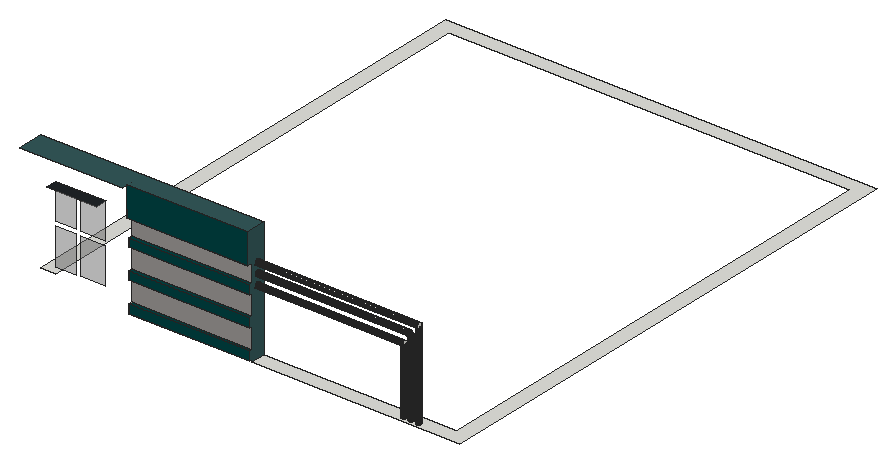
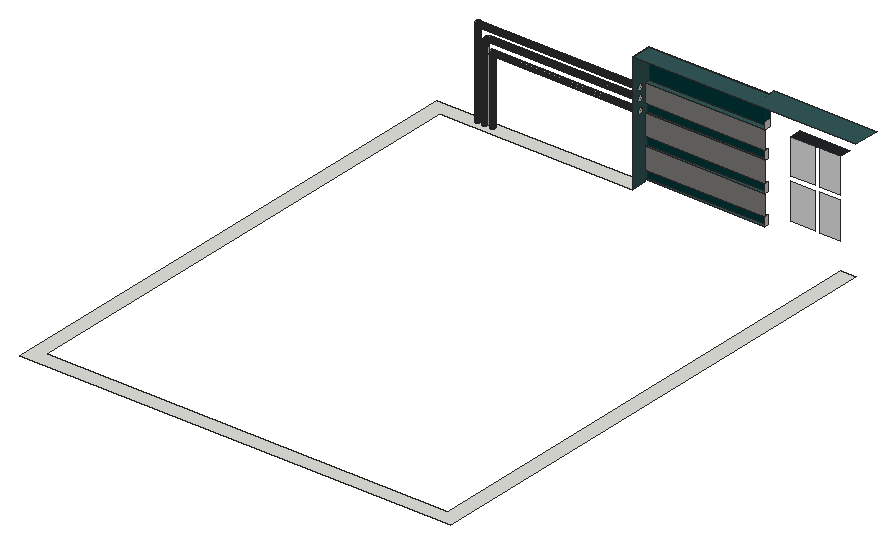
# SketchUp Ruby script. Lengths in inches.
U = 1.inch
M = Sketchup.active_model
def pt(a) = Geom::Point3d.new(a.map { |v| v * U })
def face(e, loops, mat)
  f = e.add_face(loops[0].map { |a| pt(a) })
  loops[1..].each { |l| e.add_face(l.map { |a| pt(a) }).erase! }
  f.material = f.back_material = mat if mat
  f
end
# faces: each face lists its corners as indices into pts; further lists are holes
def faces(e, pts, list, mat = nil) = list.each { |f| face(e, (f[0].is_a?(Array) ? f : [f]).map { |l| l.map { |i| pts[i] } }, mat) }
# xy, xz, yz: faces in a plane at the given z, y or x. An outline is a flat list of corners, or four numbers for a rectangle; further outlines are holes
def ring(l) = l.size == 4 ? [[l[0], l[1]], [l[2], l[1]], [l[2], l[3]], [l[0], l[3]]] : l.each_slice(2).to_a
def flat(e, list, mat, &to3) = list.each { |f| face(e, (f[0].is_a?(Array) ? f : [f]).map { |l| ring(l).map { |u, v| to3.(u, v) } }, mat) }
def xy(e, z, list, mat = nil) = flat(e, list, mat) { |x, y| [x, y, z] }
def xz(e, y, list, mat = nil) = flat(e, list, mat) { |x, z| [x, y, z] }
def yz(e, x, list, mat = nil) = flat(e, list, mat) { |y, z| [x, y, z] }
def lines(e, pts, list) = list.each { |a, b| e.add_line(pt(pts[a]), pt(pts[b])) }
# prism: a flat outline (further loops are holes) pulled along v
def prism(e, loops, v, mat = nil)
  f = face(e, loops, mat); d = Geom::Vector3d.new(v.map { |x| x * U })
  f.pushpull(f.normal.samedirection?(d) ? d.length : -d.length)
end
def box(e, o, s, mat = nil) = prism(e, [[o, [o[0] + s[0], o[1], o[2]], [o[0] + s[0], o[1] + s[1], o[2]], [o[0], o[1] + s[1], o[2]]]], [0, 0, s[2]], mat)
def at(x, y, z, deg = 0) = Geom::Transformation.translation(pt([x, y, z])) * Geom::Transformation.rotation(ORIGIN, Z_AXIS, deg.degrees)
def axes(o, x, y, z) = Geom::Transformation.new([*x, 0, *y, 0, *z, 0, *pt(o).to_a, 1])
def part(name) = M.definitions.add(name)
# library, detail: a bought-in or finely detailed component or shape, given as its bounding box
def library(name, o, s) = part(name).tap { |d| box(d.entities, o, s) }
def detail(e, o, s) = box(e.add_group.entities, o, s)
def put(e, d, t, mat = nil) = e.add_instance(d, t).tap { |i| i.material = mat if mat }
def group(e, t, mat = nil) = e.add_group.tap { |g| g.transformation = t; g.material = mat if mat }.entities
root = M.entities
M.materials.add("[0079_Teal]").color = [0, 66, 66]
M.materials.add("[0081_CadetBlue]1").color = [52, 88, 89]
M.materials.add("[0099_LightSteelBlue]").color = [32, 36, 40]
M.materials.add("[Concrete Aggregate Smoke]").color = [154, 150, 148]
M.materials.add("[Translucent Glass Gray]").color = [128, 128, 128]
M.materials["[Translucent Glass Gray]"].alpha = 0.5
xy(root,276,[[[180,60,348,60,348,480,0,480,0,72,12,72,12,468,336,468,336,72,180,72],[311.224,62.569,310.702,62.579,310.2,62.725,309.754,62.995,309.392,63.372,309.14,63.829,309.016,64.336,309.026,64.858,309.172,65.36,309.442,65.806,309.819,66.168,310.276,66.42,310.783,66.544,311.305,66.534,311.806,66.388,312.253,66.118,312.615,65.741,312.866,65.284,312.991,64.777,312.98,64.255,312.835,63.754,312.565,63.307,312.188,62.945,311.731,62.694],[305.224,62.569,304.702,62.579,304.2,62.725,303.754,62.995,303.392,63.372,303.14,63.829,303.016,64.336,303.026,64.858,303.172,65.36,303.442,65.806,303.819,66.168,304.276,66.42,304.783,66.544,305.305,66.534,305.806,66.388,306.253,66.118,306.615,65.741,306.866,65.284,306.991,64.777,306.98,64.255,306.835,63.754,306.565,63.307,306.188,62.945,305.731,62.694],[299.224,62.569,298.702,62.579,298.2,62.725,297.754,62.995,297.392,63.372,297.14,63.829,297.016,64.336,297.026,64.858,297.172,65.36,297.442,65.806,297.819,66.168,298.276,66.42,298.783,66.544,299.305,66.534,299.806,66.388,300.253,66.118,300.615,65.741,300.866,65.284,300.991,64.777,300.98,64.255,300.835,63.754,300.565,63.307,300.188,62.945,299.731,62.694]],[299.224,62.569,298.702,62.579,298.2,62.725,297.754,62.995,297.392,63.372,297.14,63.829,297.016,64.336,297.026,64.858,297.172,65.36,297.442,65.806,297.819,66.168,298.276,66.42,298.783,66.544,299.305,66.534,299.806,66.388,300.253,66.118,300.615,65.741,300.866,65.284,300.991,64.777,300.98,64.255,300.835,63.754,300.565,63.307,300.188,62.945,299.731,62.694],[305.224,62.569,304.702,62.579,304.2,62.725,303.754,62.995,303.392,63.372,303.14,63.829,303.016,64.336,303.026,64.858,303.172,65.36,303.442,65.806,303.819,66.168,304.276,66.42,304.783,66.544,305.305,66.534,305.806,66.388,306.253,66.118,306.615,65.741,306.866,65.284,306.991,64.777,306.98,64.255,306.835,63.754,306.565,63.307,306.188,62.945,305.731,62.694],[311.224,62.569,310.702,62.579,310.2,62.725,309.754,62.995,309.392,63.372,309.14,63.829,309.016,64.336,309.026,64.858,309.172,65.36,309.442,65.806,309.819,66.168,310.276,66.42,310.783,66.544,311.305,66.534,311.806,66.388,312.253,66.118,312.615,65.741,312.866,65.284,312.991,64.777,312.98,64.255,312.835,63.754,312.565,63.307,312.188,62.945,311.731,62.694]])
xy(root,278.155,[[82.708,57.5,180,60]],"[0081_CadetBlue]1")
xy(root,285.216,[[82.708,57.5,180,60]],"[0079_Teal]")
xy(root,302.155,[[82.708,57.5,180,60]],"[0081_CadetBlue]1")
xy(root,309.216,[[82.708,57.5,180,60]],"[0079_Teal]")
xy(root,326.155,[[82.708,57.5,180,60]],"[0081_CadetBlue]1")
xy(root,329.8125,[[299.224,62.569,299.731,62.694,300.188,62.945,300.565,63.307,300.835,63.754,300.98,64.255,300.991,64.777,300.866,65.284,300.615,65.741,300.253,66.118,299.806,66.388,299.305,66.534,298.783,66.544,298.276,66.42,297.819,66.168,297.442,65.806,297.172,65.36,297.026,64.858,297.02,64.557,297.016,64.336,297.14,63.829,297.392,63.372,297.754,62.995,298.2,62.725,298.702,62.579]])
xy(root,333.216,[[82.708,57.5,180,60]],"[0079_Teal]")
xy(root,346.75,[[311.224,62.569,311.731,62.694,312.188,62.945,312.565,63.307,312.835,63.754,312.98,64.255,312.991,64.777,312.866,65.284,312.615,65.741,312.253,66.118,311.806,66.388,311.305,66.534,310.783,66.544,310.276,66.42,309.819,66.168,309.442,65.806,309.172,65.36,309.026,64.858,309.02,64.557,309.016,64.336,309.14,63.829,309.392,63.372,309.754,62.995,310.2,62.725,310.702,62.579]])
xy(root,348,[[82.708,55.5,180,60]],"[0081_CadetBlue]1")
xy(root,350.786,[[21.214,51,61.494,60]],"[0099_LightSteelBlue]")
xy(root,372,[[0,51,82.708,51,82.708,55.5,180,55.5,180,72,0,72]],"[0081_CadetBlue]1")
xz(root,55.5,[[82.708,348,180,372]],"[0079_Teal]")
xz(root,57.5,[[82.708,278.155,180,285.216],[82.708,302.155,180,309.216],[82.708,326.155,180,333.216]],"[0079_Teal]")
xz(root,60,[[82.708,285.216,180,302.155],[82.708,309.216,180,326.155],[82.708,333.216,180,348]],"[Concrete Aggregate Smoke]")
xz(root,60,[[21.214,288.791,38.354,318.791],[41.354,288.791,61.494,318.791],[21.214,321.791,38.354,350.786],[41.354,321.791,61.494,350.786]],"[Translucent Glass Gray]")
yz(root,82.708,[[57.5,278.155,60,285.216],[57.5,302.155,60,309.216],[57.5,326.155,60,333.216],[55.5,348,60,354]])
yz(root,180,[[64.557,327.8125,64.039,327.881,63.557,328.08,63.142,328.398,62.825,328.8125,62.625,329.295,62.557,329.8125,62.625,330.33,62.825,330.8125,63.142,331.227,63.557,331.545,64.039,331.744,64.557,331.8125,65.074,331.744,65.557,331.545,65.971,331.227,66.289,330.8125,66.488,330.33,66.557,329.8125,66.488,329.295,66.289,328.8125,65.971,328.398,65.557,328.08,65.074,327.881],[64.557,336.8125,64.039,336.881,63.557,337.08,63.142,337.398,62.825,337.8125,62.625,338.295,62.557,338.8125,62.625,339.33,62.825,339.8125,63.142,340.227,63.557,340.545,64.039,340.744,64.557,340.8125,65.074,340.744,65.557,340.545,65.971,340.227,66.289,339.8125,66.488,339.33,66.557,338.8125,66.488,338.295,66.289,337.8125,65.971,337.398,65.557,337.08,65.074,336.881],[64.557,344.75,64.039,344.818,63.557,345.018,63.142,345.336,62.825,345.75,62.625,346.232,62.557,346.75,62.625,347.268,62.825,347.75,63.142,348.164,63.557,348.482,64.039,348.682,64.557,348.75,65.074,348.682,65.557,348.482,65.971,348.164,66.289,347.75,66.488,347.268,66.557,346.75,66.488,346.232,66.289,345.75,65.971,345.336,65.557,345.018,65.074,344.818]])
yz(root,180,[[[60,276,72,276,72,372,55.5,372,55.5,348,60,348,60,333.216,57.5,333.216,57.5,326.155,60,326.155,60,309.216,57.5,309.216,57.5,302.155,60,302.155,60,285.216,57.5,285.216,57.5,278.155,60,278.155],[64.557,327.8125,64.039,327.881,63.557,328.08,63.142,328.398,62.825,328.8125,62.625,329.295,62.557,329.8125,62.625,330.33,62.825,330.8125,63.142,331.227,63.557,331.545,64.039,331.744,64.557,331.8125,65.074,331.744,65.557,331.545,65.971,331.227,66.289,330.8125,66.488,330.33,66.557,329.8125,66.488,329.295,66.289,328.8125,65.971,328.398,65.557,328.08,65.074,327.881],[64.557,344.75,64.039,344.818,63.557,345.018,63.142,345.336,62.825,345.75,62.625,346.232,62.557,346.75,62.625,347.268,62.825,347.75,63.142,348.164,63.557,348.482,64.039,348.682,64.557,348.75,65.074,348.682,65.557,348.482,65.971,348.164,66.289,347.75,66.488,347.268,66.557,346.75,66.488,346.232,66.289,345.75,65.971,345.336,65.557,345.018,65.074,344.818],[64.557,336.8125,64.039,336.881,63.557,337.08,63.142,337.398,62.825,337.8125,62.625,338.295,62.557,338.8125,62.625,339.33,62.825,339.8125,63.142,340.227,63.557,340.545,64.039,340.744,64.557,340.8125,65.074,340.744,65.557,340.545,65.971,340.227,66.289,339.8125,66.488,339.33,66.557,338.8125,66.488,338.295,66.289,337.8125,65.971,337.398,65.557,337.08,65.074,336.881]]],"[0081_CadetBlue]1")
yz(root,300.083,[[64.557,327.8125,65.074,327.881,65.557,328.08,65.971,328.398,66.289,328.8125,66.488,329.295,66.557,329.8125,66.488,330.33,66.289,330.8125,65.971,331.227,65.557,331.545,65.074,331.744,64.557,331.8125,64.039,331.744,63.557,331.545,63.142,331.227,62.825,330.8125,62.625,330.33,62.557,329.8125,62.625,329.295,62.825,328.8125,63.142,328.398,63.557,328.08,64.039,327.881]])
yz(root,301.303,[[64.557,336.8125,65.074,336.881,65.557,337.08,65.971,337.398,66.289,337.8125,66.488,338.295,66.557,338.8125,66.488,339.33,66.289,339.8125,65.971,340.227,65.557,340.545,65.074,340.744,64.557,340.8125,64.039,340.744,63.557,340.545,63.142,340.227,62.825,339.8125,62.625,339.33,62.557,338.8125,62.625,338.295,62.825,337.8125,63.142,337.398,63.557,337.08,64.039,336.881]])
yz(root,312.02,[[64.557,344.75,65.074,344.818,65.557,345.018,65.971,345.336,66.289,345.75,66.488,346.232,66.557,346.75,66.488,347.268,66.289,347.75,65.971,348.164,65.557,348.482,65.074,348.682,64.557,348.75,64.039,348.682,63.557,348.482,63.142,348.164,62.825,347.75,62.625,347.268,62.557,346.75,62.625,346.232,62.825,345.75,63.142,345.336,63.557,345.018,64.039,344.818]])
p = [[298.2,62.725,276],[298.702,62.579,276],[298.702,62.579,329.8125],[298.2,62.725,329.8125],[299.224,62.569,276],[299.224,62.569,329.8125],
  [299.731,62.694,276],[299.731,62.694,329.8125],[304.2,62.725,276],[304.702,62.579,276],[304.702,62.58,335.093],[304.702,62.579,335.113],
  [304.2,62.725,335.113],[305.224,62.569,276],[305.224,62.569,335.113],[305.003,62.573,335.113],[305.731,62.694,276],[305.731,62.694,335.113],
  [310.2,62.725,276],[310.702,62.579,276],[310.702,62.579,346.75],[310.2,62.725,346.75],[311.224,62.569,276],[311.224,62.569,346.75],
  [311.731,62.694,276],[311.731,62.694,346.75],[297.754,62.995,276],[297.754,62.995,329.8125],[300.188,62.945,276],[300.188,62.945,329.8125],
  [303.754,62.995,276],[303.754,62.995,335.113],[306.188,62.945,276],[306.188,62.945,335.113],[309.754,62.995,276],[309.754,62.995,346.75],
  [312.188,62.945,276],[312.188,62.945,346.75],[300.565,63.307,276],[300.565,63.307,329.8125],[306.565,63.307,276],[306.565,63.307,335.113],
  [312.565,63.307,276],[312.565,63.307,346.75],[297.392,63.372,276],[297.392,63.372,329.8125],[303.392,63.372,276],[303.392,63.372,335.113],
  [309.392,63.372,276],[309.392,63.372,346.75],[300.835,63.754,276],[300.835,63.754,329.8125],[306.835,63.754,276],[306.835,63.754,335.113],
  [312.835,63.754,276],[312.835,63.754,346.75],[297.14,63.829,276],[297.14,63.829,329.8125],[303.14,63.829,276],[303.14,63.829,335.113],
  [309.14,63.829,276],[309.14,63.829,346.75],[297.016,64.336,276],[297.016,64.336,329.8125],[300.98,64.255,276],[300.98,64.255,329.8125],
  [303.016,64.336,276],[303.016,64.336,335.113],[306.98,64.255,276],[306.98,64.255,335.113],[309.016,64.336,276],[309.016,64.336,346.75],
  [312.98,64.255,276],[312.98,64.255,346.75],[297.026,64.858,276],[297.02,64.557,329.8125],[297.026,64.858,329.8125],[300.991,64.777,276],
  [300.991,64.777,329.8125],[303.026,64.858,276],[303.026,64.858,335.113],[306.991,64.777,276],[306.991,64.777,335.113],[309.026,64.858,276],
  [309.02,64.557,346.75],[309.026,64.858,346.75],[312.991,64.777,276],[312.991,64.777,346.75],[300.866,65.284,276],[300.866,65.284,329.8125],
  [306.866,65.284,276],[306.866,65.284,335.113],[312.866,65.284,276],[312.866,65.284,346.75],[297.172,65.36,276],[297.172,65.36,329.8125],
  [303.172,65.36,276],[303.172,65.36,335.113],[309.172,65.36,276],[309.172,65.36,346.75],[300.615,65.741,276],[300.615,65.741,329.8125],
  [306.615,65.741,276],[306.615,65.741,335.113],[312.615,65.741,276],[312.615,65.741,346.75],[297.442,65.806,276],[297.442,65.806,329.8125],
  [303.442,65.806,276],[303.442,65.806,335.113],[309.442,65.806,276],[309.442,65.806,346.75],[300.253,66.118,276],[300.253,66.118,329.8125],
  [306.253,66.118,276],[306.253,66.118,335.113],[312.253,66.118,276],[312.253,66.118,346.75],[297.819,66.168,276],[297.819,66.168,329.8125],
  [303.819,66.168,276],[303.819,66.168,335.113],[309.819,66.168,276],[309.819,66.168,346.75],[299.806,66.388,276],[299.806,66.388,329.8125],
  [305.806,66.388,276],[305.806,66.388,335.113],[311.806,66.388,276],[311.806,66.388,346.75],[298.276,66.42,276],[298.276,66.42,329.8125],
  [304.276,66.42,276],[304.276,66.42,335.113],[310.276,66.42,276],[310.276,66.42,346.75],[298.783,66.544,276],[298.783,66.544,329.8125],
  [299.305,66.534,276],[299.305,66.534,329.8125],[304.783,66.544,276],[304.783,66.544,335.113],[304.784,66.544,335.098],[305.305,66.534,276],
  [305.305,66.534,335.113],[310.783,66.544,276],[310.783,66.544,346.75],[311.305,66.534,276],[311.305,66.534,346.75],[305.003,66.54,335.113],
  [180,64.039,327.881],[180,64.557,327.8125],[299.003,64.557,327.8125],[300.083,64.557,327.8125],[300.083,64.039,327.881],[180,65.074,327.881],
  [300.083,65.074,327.881],[180,63.557,328.08],[300.083,63.557,328.08],[180,65.557,328.08],[300.083,65.557,328.08],[180,63.142,328.398],
  [300.083,63.142,328.398],[180,65.971,328.398],[300.083,65.971,328.398],[180,62.825,328.8125],[300.083,62.825,328.8125],[180,66.289,328.8125],
  [300.083,66.289,328.8125],[180,62.625,329.295],[300.083,62.625,329.295],[180,66.488,329.295],[300.083,66.488,329.295],[180,62.557,329.8125],
  [300.083,62.557,329.8125],[180,66.557,329.8125],[300.083,66.557,329.8125],[180,62.625,330.33],[300.083,62.625,330.33],[180,66.488,330.33],
  [300.083,66.488,330.33],[180,62.825,330.8125],[300.083,62.825,330.8125],[180,66.289,330.8125],[300.083,66.289,330.8125],[180,63.142,331.227],
  [300.083,63.142,331.227],[180,65.971,331.227],[300.083,65.971,331.227],[180,63.557,331.545],[300.083,63.557,331.545],[180,65.557,331.545],
  [300.083,65.557,331.545],[180,64.039,331.744],[300.083,64.039,331.744],[180,65.074,331.744],[300.083,65.074,331.744],[180,64.557,331.8125],
  [300.083,64.557,331.8125],[306.608,65.741,335.218],[306.858,65.284,335.234],[306.983,64.777,335.242],[306.972,64.255,335.242],[306.827,63.754,335.232],
  [306.558,63.307,335.214],[306.183,62.945,335.19],[305.728,62.694,335.16],[305.223,62.569,335.127],[304.703,62.579,335.093],[304.204,62.725,335.06],
  [303.759,62.995,335.031],[303.399,63.372,335.007],[303.148,63.829,334.991],[303.024,64.336,334.983],[303.035,64.858,334.983],[303.179,65.36,334.993],
  [303.449,65.806,335.011],[303.824,66.168,335.035],[304.279,66.42,335.065],[305.304,66.534,335.132],[305.803,66.388,335.165],[306.248,66.118,335.194],
  [304.673,62.579,335.556],[304.176,62.725,335.491],[305.19,62.569,335.624],[305.693,62.694,335.69],[303.733,62.995,335.432],[303.374,63.372,335.385],
  [303.125,63.829,335.352],[303.001,64.336,335.336],[303.011,64.858,335.337],[303.156,65.36,335.356],[303.424,65.806,335.392],[303.797,66.168,335.441],
  [304.251,66.42,335.501],[304.753,66.544,335.567],[305.271,66.534,335.635],[305.768,66.388,335.7],[306.146,62.945,335.75],[306.52,63.307,335.799],
  [306.788,63.754,335.835],[306.932,64.255,335.854],[306.943,64.777,335.855],[306.819,65.284,335.839],[306.569,65.741,335.806],[306.211,66.118,335.759],
  [303.078,63.829,335.588],[302.957,64.336,335.556],[302.968,64.858,335.558],[303.108,65.36,335.596],[304.102,62.725,335.862],[303.67,62.995,335.747],
  [303.321,63.372,335.653],[303.369,65.806,335.666],[303.733,66.168,335.763],[304.175,66.42,335.882],[304.586,62.579,335.992],[304.664,66.544,336.013],
  [305.09,62.569,336.127],[305.58,62.694,336.258],[303.233,63.372,335.912],[303,63.829,335.815],[302.885,64.336,335.768],[302.895,64.858,335.772],
  [303.029,65.36,335.827],[303.279,65.806,335.931],[305.169,66.534,336.148],[305.653,66.388,336.278],[303.98,62.725,336.221],[303.567,62.995,336.05],
  [306.022,62.945,336.377],[303.627,66.168,336.075],[306.084,66.118,336.394],[306.386,63.307,336.474],[306.647,63.754,336.544],[303.112,63.372,336.157],
  [302.894,63.829,336.031],[302.786,64.336,335.969],[306.787,64.255,336.582],[302.795,64.858,335.974],[306.677,65.284,336.552],[306.797,64.777,336.585],
  [302.921,65.36,336.047],[306.434,65.741,336.487],[303.155,65.806,336.182],[304.05,66.42,336.25],[304.443,62.579,336.413],[303.425,62.995,336.338],
  [303.482,66.168,336.37],[304.518,66.544,336.444],[304.925,62.569,336.613],[302.96,63.372,336.384],[302.761,63.829,336.231],[302.662,64.336,336.155],
  [302.67,64.858,336.161],[302.786,65.36,336.25],[303,65.806,336.414],[305,66.534,336.644],[305.394,62.694,336.807],[303.812,62.725,336.561],
  [303.878,66.42,336.599],[305.464,66.388,336.836],[304.246,62.579,336.812],[303.247,62.995,336.604],[302.78,63.372,336.589],[302.602,63.829,336.411],
  [302.514,64.336,336.323],[302.522,64.858,336.331],[302.624,65.36,336.434],[302.816,65.806,336.625],[303.299,66.168,336.644],[303.602,62.725,336.876],
  [305.816,62.945,336.982],[302.422,63.829,336.57],[302.346,64.336,336.471],[302.352,64.858,336.479],[302.441,65.36,336.595],[305.876,66.118,337.007],
  [304.317,66.544,336.852],[304.699,62.569,337.073],[306.164,63.307,337.126],[303.036,62.995,336.845],[302.575,63.372,336.77],[302.605,65.806,336.809],
  [306.21,65.741,337.145],[303.082,66.168,336.891],[303.662,66.42,336.922],[304.769,66.534,337.113],[306.414,63.754,337.229],[302.222,63.829,336.703],
  [302.159,64.336,336.595],[306.548,64.255,337.285],[302.165,64.858,336.605],[302.238,65.36,336.731],[306.443,65.284,337.241],[303.999,62.579,337.181],
  [305.138,62.694,337.326],[303.352,62.725,337.161],[302.795,62.995,337.056],[302.348,63.372,336.921],[302.006,63.829,336.81],[301.959,64.336,336.694],
  [301.963,64.858,336.704],[306.558,64.777,337.289],[302.018,65.36,336.839],[302.373,65.806,336.965],[302.835,66.168,337.108],[303.405,66.42,337.214],
  [304.064,66.544,337.231],[305.203,66.388,337.364],[302.103,63.372,337.042],[301.779,63.829,336.887],[301.746,64.336,336.766],[301.749,64.858,336.777],
  [301.787,65.36,336.917],[302.122,65.806,337.088],[301.425,65.284,340.668],[301.409,65.741,340.417],[301.385,66.118,340.057],[301.356,66.388,339.612],
  [301.323,66.534,339.113],[301.289,66.544,338.593],[301.256,66.42,338.088],[301.226,66.168,337.633],[301.201,65.806,337.258],[301.184,65.36,336.989],
  [301.174,64.858,336.844],[301.174,64.336,336.833],[301.182,63.829,336.957],[301.198,63.372,337.208],[301.222,62.995,337.568],[301.251,62.725,338.013],
  [301.284,62.579,338.512],[301.318,62.569,339.032],[301.351,62.694,339.537],[301.381,62.945,339.992],[301.405,63.307,340.367],[301.423,63.754,340.636],
  [301.432,64.255,340.781],[301.433,64.777,340.792],[304.414,62.569,337.499],[303.067,62.725,337.411],[305.534,62.945,337.555],[302.528,62.995,337.234],
  [301.844,63.372,337.13],[301.527,64.336,336.81],[301.543,63.829,336.934],[180,64.039,336.881],[180,64.557,336.8125],[301.303,64.557,336.8125],
  [301.303,64.039,336.881],[301.528,64.858,336.821],[180,65.074,336.881],[301.303,65.074,336.881],[301.547,65.36,336.965],[301.857,65.806,337.178],
  [302.561,66.168,337.291],[305.59,66.118,337.587],[303.706,62.579,337.516],[302.241,62.995,337.376],[301.576,63.372,337.183],[180,63.557,337.08],
  [301.303,63.557,337.08],[180,65.557,337.08],[301.303,65.557,337.08],[301.582,65.806,337.233],[303.113,66.42,337.471],[303.764,66.544,337.573],
  [304.478,66.534,337.549],[305.86,63.307,337.743],[301.9375,62.995,337.479],[305.903,65.741,337.768],[302.266,66.168,337.436],[304.816,62.694,337.808],
  [302.752,62.725,337.621],[301.623,62.995,337.542],[180,63.142,337.398],[301.303,63.142,337.398],[306.094,63.754,337.878],[306.121,65.284,337.894],
  [180,65.971,337.398],[301.303,65.971,337.398],[301.954,66.168,337.542],[302.79,66.42,337.687],[304.876,66.388,337.854],[303.372,62.579,337.809],
  [304.075,62.569,337.885],[302.412,62.725,337.789],[306.22,64.255,337.951],[306.229,64.777,337.956],[301.632,66.168,337.606],[303.422,66.544,337.873],
  [304.133,66.534,337.942],[305.179,62.945,338.086],[302.441,66.42,337.859],[303.003,62.579,338.056],[302.053,62.725,337.911],[180,62.825,337.8125],
  [301.303,62.825,337.8125],[180,66.289,337.8125],[301.303,66.289,337.8125],[305.23,66.118,338.126],[302.073,66.42,337.984],[303.69,62.569,338.223],
  [304.434,62.694,338.243],[301.681,62.725,337.985],[301.691,66.42,338.06],[303.043,66.544,338.126],[304.487,66.388,338.297],[302.604,62.579,338.252],
  [305.478,63.307,338.315],[305.517,65.741,338.346],[303.739,66.534,338.287],[305.692,63.754,338.48],[302.635,66.544,338.327],[180,62.625,338.295],
  [301.303,62.625,338.295],[302.183,62.579,338.395],[303.264,62.569,338.508],[304.757,62.945,338.567],[305.717,65.284,338.499],[180,66.488,338.295],
  [301.303,66.488,338.295],[301.747,62.579,338.482],[303.999,62.694,338.625],[305.807,64.255,338.569],[305.816,64.777,338.575],[304.803,66.118,338.613],
  [302.204,66.544,338.474],[304.045,66.388,338.685],[303.304,66.534,338.578],[301.758,66.544,338.5625],[302.804,62.569,338.734],[305.024,63.307,338.833],
  [305.059,65.741,338.868],[302.835,66.534,338.81],[303.517,62.694,338.947],[304.277,62.945,338.988],[180,62.557,338.8125],[301.303,62.557,338.8125],
  [302.318,62.569,338.899],[305.215,63.754,339.024],[305.237,65.284,339.046],[304.317,66.118,339.039],[303.555,66.388,339.012],[180,66.557,338.8125],
  [301.303,66.557,338.8125],[302.339,66.534,338.978],[301.815,62.569,338.999],[302.998,62.694,339.203],[305.318,64.255,339.127],[305.325,64.777,339.134],
  [301.826,66.534,339.08],[303.746,62.945,339.343],[304.506,63.307,339.287],[304.537,65.741,339.326],[303.027,66.388,339.273],[302.449,62.694,339.389],
  [303.778,66.118,339.399],[180,62.625,339.33],[301.303,62.625,339.33],[304.671,63.754,339.501],[302.469,66.388,339.462],[180,66.488,339.33],
  [301.303,66.488,339.33],[301.881,62.694,339.502],[303.173,62.945,339.625],[304.69,65.284,339.526],[303.934,63.307,339.669],[304.759,64.255,339.616],
  [304.766,64.777,339.625],[303.959,65.741,339.712],[303.198,66.118,339.685],[301.891,66.388,339.577],[302.568,62.945,339.831],[180,62.825,339.8125],
  [301.303,62.825,339.8125],[303.317,63.307,339.973],[304.069,63.754,339.903],[304.085,65.284,339.93],[302.584,66.118,339.894],[180,66.289,339.8125],
  [301.303,66.289,339.8125],[301.941,62.945,339.955],[303.336,65.741,340.02],[304.142,64.255,340.029],[304.147,64.777,340.038],[301.949,66.118,340.02],
  [302.665,63.307,340.195],[303.42,63.754,340.223],[303.432,65.284,340.252],[302.678,65.741,340.243],[180,63.142,340.227],[301.303,63.142,340.227],
  [301.99,63.307,340.329],[180,65.971,340.227],[301.303,65.971,340.227],[303.476,64.255,340.357],[303.48,64.777,340.367],[301.997,65.741,340.378],
  [302.735,63.754,340.456],[302.743,65.284,340.486],[180,63.557,340.545],[301.303,63.557,340.545],[302.025,63.754,340.597],[302.773,64.255,340.596],
  [302.029,65.284,340.628],[180,65.557,340.545],[301.303,65.557,340.545],[302.775,64.777,340.607],[180,64.039,340.744],[301.303,64.039,340.744],
  [302.044,64.255,340.741],[302.046,64.777,340.752],[180,65.074,340.744],[301.303,65.074,340.744],[180,64.557,340.8125],[301.303,64.557,340.8125],
  [180,64.039,344.818],[180,64.557,344.75],[311.003,64.557,344.75],[312.02,64.557,344.75],[312.02,64.039,344.818],[180,65.074,344.818],
  [312.02,65.074,344.818],[180,63.557,345.018],[312.02,63.557,345.018],[180,65.557,345.018],[312.02,65.557,345.018],[180,63.142,345.336],
  [312.02,63.142,345.336],[180,65.971,345.336],[312.02,65.971,345.336],[180,62.825,345.75],[312.02,62.825,345.75],[180,66.289,345.75],
  [312.02,66.289,345.75],[180,62.625,346.232],[312.02,62.625,346.232],[180,66.488,346.232],[312.02,66.488,346.232],[180,62.557,346.75],
  [312.02,62.557,346.75],[180,66.557,346.75],[312.02,66.557,346.75],[180,62.625,347.268],[312.02,62.625,347.268],[180,66.488,347.268],
  [312.02,66.488,347.268],[180,62.825,347.75],[312.02,62.825,347.75],[180,66.289,347.75],[312.02,66.289,347.75],[180,63.142,348.164],
  [312.02,63.142,348.164],[180,65.971,348.164],[312.02,65.971,348.164],[180,63.557,348.482],[312.02,63.557,348.482],[180,65.557,348.482],
  [312.02,65.557,348.482],[180,64.039,348.682],[312.02,64.039,348.682],[180,65.074,348.682],[312.02,65.074,348.682],[180,64.557,348.75],
  [312.02,64.557,348.75],[82.708,60,372],[82.708,60,354],[311.003,64.557,276],[311.003,64.557,346.75],[305.003,64.557,276],
  [305.003,64.557,335.113],[299.003,64.557,276],[299.003,64.557,329.8125],[180,64.557,346.75],[301.303,64.557,338.8125],[301.786,64.557,338.781],
  [302.261,64.557,338.686],[302.719,64.557,338.531],[303.153,64.557,338.317],[303.556,64.557,338.048],[303.92,64.557,337.729],[304.239,64.557,337.365],
  [304.508,64.557,336.963],[304.722,64.557,336.528],[304.877,64.557,336.07],[304.972,64.557,335.595],[180,64.557,338.8125],[180,64.557,329.8125]]
faces(root,p,[[0,1,2,3],[1,4,5,2],[4,6,7,5],[8,9,10,11,12],[9,13,14,15,11,10],[13,16,17,14],[18,19,20,21],[19,22,23,20],
  [22,24,25,23],[26,0,3,27],[6,28,29,7],[30,8,12,31],[16,32,33,17],[34,18,21,35],[24,36,37,25],[28,38,39,29],
  [32,40,41,33],[36,42,43,37],[44,26,27,45],[46,30,31,47],[48,34,35,49],[38,50,51,39],[40,52,53,41],[42,54,55,43],
  [56,44,45,57],[58,46,47,59],[60,48,49,61],[62,56,57,63],[50,64,65,51],[66,58,59,67],[52,68,69,53],[70,60,61,71],
  [54,72,73,55],[74,62,63,75,76],[64,77,78,65],[79,66,67,80],[68,81,82,69],[83,70,71,84,85],[72,86,87,73],[77,88,89,78],
  [81,90,91,82],[86,92,93,87],[94,74,76,95],[96,79,80,97],[98,83,85,99],[88,100,101,89],[90,102,103,91],[92,104,105,93],
  [106,94,95,107],[108,96,97,109],[110,98,99,111],[100,112,113,101],[102,114,115,103],[104,116,117,105],[118,106,107,119],[120,108,109,121],
  [122,110,111,123],[112,124,125,113],[114,126,127,115],[116,128,129,117],[130,118,119,131],[132,120,121,133],[134,122,123,135],[136,130,131,137],
  [124,138,139,125],[140,132,133,141,142],[126,143,144,127],[145,134,135,146],[128,147,148,129],[138,136,137,139],[140,142,149,144,143],[147,145,146,148],
  [150,151,152,153,154],[151,155,156,153,152],[157,150,154,158],[155,159,160,156],[161,157,158,162],[159,163,164,160],[165,161,162,166],[163,167,168,164],
  [169,165,166,170],[167,171,172,168],[173,169,170,174],[171,175,176,172],[177,173,174,178],[175,179,180,176],[181,177,178,182],[179,183,184,180],
  [185,181,182,186],[183,187,188,184],[189,185,186,190],[187,191,192,188],[193,189,190,194],[191,195,196,192],[197,193,194,198],[195,197,198,196],
  [199,200,201,202,203,204,205,206,207,15,208,10,209,210,211,212,213,214,215,216,217,218,142,149,219,220,221],[209,12,31,210],[210,31,47,211],[211,47,59,212],[212,59,67,213],[213,67,80,214],[214,80,97,215],[215,97,109,216],
  [216,109,121,217],[217,121,133,218],[209,10,208,11,222,223,12],[208,15,11],[222,11,15,207,224],[207,206,225,224],[226,31,12,223],[227,47,31,226],
  [228,59,47,227],[229,67,59,228],[230,80,67,229],[231,97,80,230],[232,109,97,231],[233,121,109,232],[234,133,121,233],[218,133,141,142],
  [235,141,133,234],[220,219,236,237],[142,141,149],[219,149,141,235,236],[206,205,238,225],[205,204,239,238],[204,203,240,239],[203,202,241,240],
  [202,201,242,241],[201,200,243,242],[200,199,244,243],[199,221,245,244],[221,220,237,245],[229,228,246,247],[230,229,247,248],[231,230,248,249],
  [226,223,250,251],[227,226,251,252],[228,227,252,246],[232,231,249,253],[233,232,253,254],[234,233,254,255],[223,222,256,250],[235,234,255,257],
  [222,224,258,256],[224,225,259,258],[246,252,260,261],[247,246,261,262],[248,247,262,263],[249,248,263,264],[253,249,264,265],[237,236,266,267],
  [236,235,257,266],[251,250,268,269],[225,238,270,259],[252,251,269,260],[254,253,265,271],[245,237,267,272],[238,239,273,270],[239,240,274,273],
  [261,260,275,276],[262,261,276,277],[240,241,278,274],[263,262,277,279],[242,243,280,281],[264,263,279,282],[243,244,283,280],[265,264,282,284],
  [244,245,272,283],[255,254,271,285],[250,256,286,268],[260,269,287,275],[241,242,281,278],[271,265,284,288],[257,255,285,289],[256,258,290,286],
  [276,275,291,292],[277,276,292,293],[279,277,293,294],[282,279,294,295],[284,282,295,296],[266,257,289,297],[258,259,298,290],[269,268,299,287],
  [285,271,288,300],[267,266,297,301],[268,286,302,299],[275,287,303,291],[292,291,304,305],[293,292,305,306],[294,293,306,307],[295,294,307,308],
  [296,295,308,309],[288,284,296,310],[287,299,311,303],[259,270,312,298],[306,305,313,314],[307,306,314,315],[308,307,315,316],[272,267,301,317],
  [289,285,300,318],[286,290,319,302],[270,273,320,312],[291,303,321,304],[305,304,322,313],[309,308,316,323],[283,272,317,324],[310,296,309,325],
  [300,288,310,326],[297,289,318,327],[273,274,328,320],[314,313,329,330],[274,278,331,328],[315,314,330,332],[316,315,332,333],[280,283,324,334],
  [299,302,335,311],[290,298,336,319],[303,311,337,321],[304,321,338,322],[313,322,339,329],[330,329,340,341],[332,330,341,342],[278,281,343,331],
  [281,280,334,343],[333,332,342,344],[323,316,333,345],[325,309,323,346],[326,310,325,347],[318,300,326,348],[301,297,327,349],[329,339,350,340],
  [341,340,351,352],[342,341,352,353],[344,342,353,354],[345,333,344,355],[356,357,358,359,360,361,362,363,364,365,366,367,368,369,370,371,372,373,374,375,376,377,378,379],[302,319,380,335],[321,337,381,338],[298,312,382,336],
  [322,338,383,339],[340,350,384,351],[385,386,368,367],[352,351,386,385],[387,388,389,390],[391,385,367,366],[353,352,385,391],[388,392,393,389],
  [394,391,366,365],[354,353,391,394],[355,344,354,395],[346,323,345,396],[317,301,349,397],[311,335,398,337],[339,383,399,350],[386,400,369,368],
  [351,384,400,386],[401,387,390,402],[392,403,404,393],[395,354,394,405],[347,325,346,406],[348,326,347,407],[327,318,348,408],[312,320,409,382],
  [350,399,410,384],[405,394,365,364],[324,317,397,411],[396,345,355,412],[319,336,413,380],[338,381,414,383],[384,410,415,400],[416,401,402,417],
  [320,328,418,409],[334,324,411,419],[403,420,421,404],[412,355,395,422],[406,346,396,423],[349,327,408,424],[337,398,425,381],[335,380,426,398],
  [383,414,427,399],[400,415,370,369],[328,331,428,418],[343,334,419,429],[430,405,364,363],[422,395,405,430],[407,347,406,431],[408,348,407,432],
  [336,382,433,413],[331,343,429,428],[423,396,412,434],[381,425,435,414],[399,427,436,410],[437,416,417,438],[420,439,440,421],[397,349,424,441],
  [434,412,422,442],[398,426,443,425],[380,413,444,426],[415,445,371,370],[410,436,445,415],[442,422,430,446],[431,406,423,447],[424,408,432,448],
  [414,435,449,427],[382,409,450,433],[411,397,441,451],[446,430,363,362],[432,407,431,452],[409,418,453,450],[447,423,434,454],[455,437,438,456],
  [427,449,457,436],[425,443,458,435],[413,433,459,444],[419,411,451,460],[439,461,462,440],[436,457,463,445],[426,444,464,443],[418,428,465,453],
  [429,419,460,466],[441,424,448,467],[454,434,442,468],[448,432,452,469],[452,431,447,470],[445,463,372,371],[428,429,466,465],[468,442,446,471],
  [435,458,472,449],[433,450,473,459],[451,441,467,474],[471,446,362,361],[470,447,454,475],[443,464,476,458],[444,459,477,464],[478,455,456,479],
  [449,472,480,457],[450,453,481,473],[460,451,474,482],[467,448,469,483],[469,452,470,484],[461,485,486,462],[475,454,468,487],[457,480,488,463],
  [463,488,373,372],[458,476,489,472],[453,465,490,481],[466,460,482,491],[487,468,471,492],[464,477,493,476],[459,473,494,477],[465,466,491,490],
  [474,467,483,495],[484,470,475,496],[492,471,361,360],[472,489,497,480],[483,469,484,498],[499,478,479,500],[473,481,501,494],[496,475,487,502],
  [485,503,504,486],[480,497,505,488],[476,493,506,489],[482,474,495,507],[488,505,374,373],[477,494,508,493],[481,490,509,501],[491,482,507,510],
  [495,483,498,511],[498,484,496,512],[502,487,492,513],[490,491,510,509],[513,492,360,359],[489,506,514,497],[515,499,500,516],[493,508,517,506],
  [494,501,518,508],[507,495,511,519],[512,496,502,520],[503,521,522,504],[497,514,523,505],[511,498,512,524],[505,523,375,374],[501,509,525,518],
  [510,507,519,526],[520,502,513,527],[506,517,528,514],[509,510,526,525],[527,513,359,358],[508,518,529,517],[519,511,524,530],[524,512,520,531],
  [532,515,516,533],[514,528,534,523],[521,535,536,522],[518,525,537,529],[526,519,530,538],[531,520,527,539],[523,534,376,375],[517,529,540,528],
  [525,526,538,537],[530,524,531,541],[539,527,358,357],[542,532,533,543],[528,540,544,534],[529,537,545,540],[541,531,539,546],[535,547,548,536],
  [534,544,377,376],[538,530,541,549],[537,538,549,545],[546,539,357,356],[550,542,543,551],[540,545,552,544],[549,541,546,553],[547,554,555,548],
  [544,552,378,377],[545,549,553,552],[553,546,356,379],[556,550,551,557],[552,553,379,378],[554,556,557,555],[558,559,560,561,562],[559,563,564,561,560],
  [565,558,562,566],[563,567,568,564],[569,565,566,570],[567,571,572,568],[573,569,570,574],[571,575,576,572],[577,573,574,578],[575,579,580,576],
  [581,577,578,582],[579,583,584,580],[585,581,582,586],[583,587,588,584],[589,585,586,590],[587,591,592,588],[593,589,590,594],[591,595,596,592],
  [597,593,594,598],[595,599,600,596],[601,597,598,602],[599,603,604,600],[605,601,602,606],[603,605,606,604]])
lines(root,p,[[607,608],[609,560],[610,84],[611,612],[613,152],[614,75],[84,615],[560,610],[616,617],[617,618],[618,619],[619,620],
  [620,621],[621,622],[622,623],[623,624],[624,625],[625,626],[626,627],[627,612],[616,628],[75,629],[152,614]])
